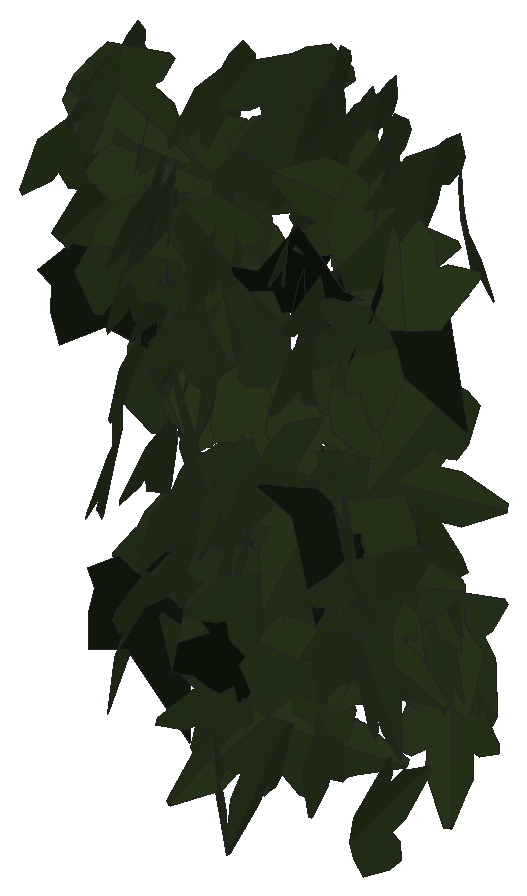
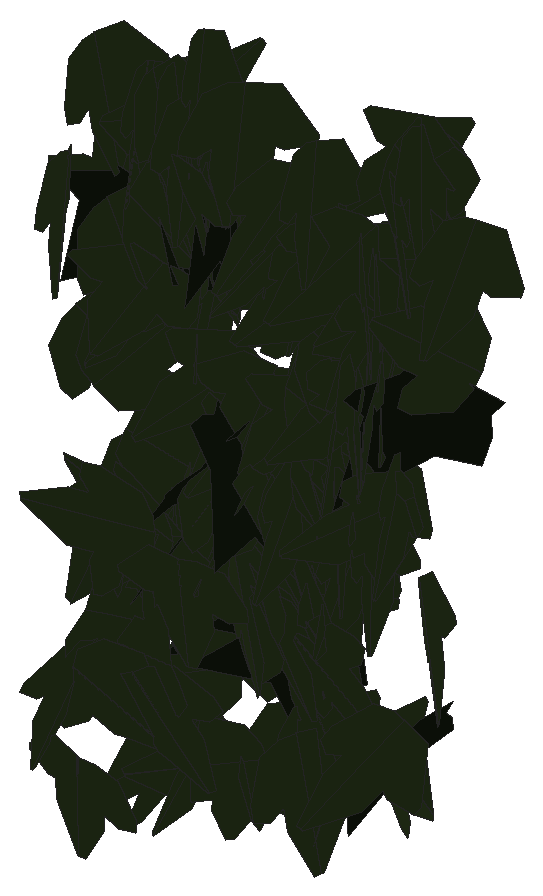
# SketchUp Ruby script. Lengths in inches.
U = 1.inch
M = Sketchup.active_model
def pt(a) = Geom::Point3d.new(a.map { |v| v * U })
def face(e, loops, mat)
  f = e.add_face(loops[0].map { |a| pt(a) })
  loops[1..].each { |l| e.add_face(l.map { |a| pt(a) }).erase! }
  f.material = f.back_material = mat if mat
  f
end
# faces: each face lists its corners as indices into pts; further lists are holes
def faces(e, pts, list, mat = nil) = list.each { |f| face(e, (f[0].is_a?(Array) ? f : [f]).map { |l| l.map { |i| pts[i] } }, mat) }
# xy, xz, yz: faces in a plane at the given z, y or x. An outline is a flat list of corners, or four numbers for a rectangle; further outlines are holes
def ring(l) = l.size == 4 ? [[l[0], l[1]], [l[2], l[1]], [l[2], l[3]], [l[0], l[3]]] : l.each_slice(2).to_a
def flat(e, list, mat, &to3) = list.each { |f| face(e, (f[0].is_a?(Array) ? f : [f]).map { |l| ring(l).map { |u, v| to3.(u, v) } }, mat) }
def xy(e, z, list, mat = nil) = flat(e, list, mat) { |x, y| [x, y, z] }
def xz(e, y, list, mat = nil) = flat(e, list, mat) { |x, z| [x, y, z] }
def yz(e, x, list, mat = nil) = flat(e, list, mat) { |y, z| [x, y, z] }
def lines(e, pts, list) = list.each { |a, b| e.add_line(pt(pts[a]), pt(pts[b])) }
# prism: a flat outline (further loops are holes) pulled along v
def prism(e, loops, v, mat = nil)
  f = face(e, loops, mat); d = Geom::Vector3d.new(v.map { |x| x * U })
  f.pushpull(f.normal.samedirection?(d) ? d.length : -d.length)
end
def box(e, o, s, mat = nil) = prism(e, [[o, [o[0] + s[0], o[1], o[2]], [o[0] + s[0], o[1] + s[1], o[2]], [o[0], o[1] + s[1], o[2]]]], [0, 0, s[2]], mat)
def at(x, y, z, deg = 0) = Geom::Transformation.translation(pt([x, y, z])) * Geom::Transformation.rotation(ORIGIN, Z_AXIS, deg.degrees)
def axes(o, x, y, z) = Geom::Transformation.new([*x, 0, *y, 0, *z, 0, *pt(o).to_a, 1])
def part(name) = M.definitions.add(name)
# library, detail: a bought-in or finely detailed component or shape, given as its bounding box
def library(name, o, s) = part(name).tap { |d| box(d.entities, o, s) }
def detail(e, o, s) = box(e.add_group.entities, o, s)
def put(e, d, t, mat = nil) = e.add_instance(d, t).tap { |i| i.material = mat if mat }
def group(e, t, mat = nil) = e.add_group.tap { |g| g.transformation = t; g.material = mat if mat }.entities
root = M.entities
M.materials.add("efeu1").color = [18, 25, 13]
M.materials.add("efeu2").color = [43, 57, 29]
c1 = part("ivyleaf_10")
p = [[0,0.5,-0.03],[-0.0625,2.02,-0.43],[-0.19,2.01,-0.46],[-0.54,1.05,-0.29],[-0.52,0.625,-0.18],[-0.83,0.76,-0.28],
  [-1.16,0.64,-0.33],[-1.15,0.33,-0.24],[-0.77,-0.39,0.02],[-0.3,-0.51,0.16],[0.04,-0.48,0.23],[-0.02,2.01,-0.4375],
  [-0.06,2.01,-0.43],[0.04,-0.49,0.23],[0.67,-0.49,0.14],[1.38,0.36,-0.2],[1.375,0.51,-0.24],[0.81,0.65,-0.19],
  [0.62,0.59,-0.15],[0.6,1.09,-0.28],[0.5,1.23,-0.31]]
faces(c1.entities,p,[[0,1,2,3,4,5,6,7,8,9,10],[11,12,0,13,14,15,16,17,18,19,20]],"efeu2")
c2 = part("ivyleaf_9")
p = [[1.54,2.16,1.25],[1.36,2.04,1.19],[-0.21,0.99,0.68],[-0.71,1.11,0.82],[-0.85,0.86,0.67],[-0.8,0.17,0.21],
  [-0.9,-0.01,0.1],[-0.67,-0.16,-0.02],[-0.08,-0.08,-0.05],[-0.03,-0.6,-0.4],[0.65,-0.88,-0.66],[0.83,-0.6,-0.49],
  [1.29,-0.42,-0.43],[1.8125,-0.07,-0.26],[1.21,0.44,0.15]]
faces(c2.entities,p,[[0,1,2,3,4,5,6,7,8,9,10,11,12,13,14]],"efeu1")
put(root,c1,axes([15.69,224.67,212.67],[-0.32703,0.04705,-0.37528],[0.36424,-0.09447,-0.32925],[-0.10189,-0.48873,0.02752]))
put(root,c1,axes([17.4,224.73,209.52],[-0.28401,-0.4041,0.07775],[-0.03453,-0.07074,-0.49377],[0.41006,-0.28584,0.01228]))
put(root,c1,axes([17.71,224.51,208.98],[-0.17834,0.44878,0.12959],[-0.06198,0.11475,-0.48269],[-0.46298,-0.18823,0.0147]))
put(root,c1,axes([15.59,224.82,212.34],[0.34047,-0.08844,0.35533],[0.34165,-0.09782,-0.35172],[0.13173,0.4823,-0.00618]))
put(root,c1,axes([14.57,224.93,213.75],[-0.00712,-0.42389,0.26508],[0.02002,-0.26514,-0.42344],[0.49955,0.00458,0.02074]))
put(root,c1,axes([17.17,224.95,213.28],[0.05774,0.30499,0.39198],[-0.05921,-0.38757,0.31029],[0.49311,-0.08225,-0.00864]))
put(root,c1,axes([15.52,224.68,210.34],[-0.34059,0.36403,-0.03849],[-0.02663,0.0278,0.49852],[0.36509,0.34163,0.00045]))
put(root,c1,axes([15.72,224.64,211.7],[-0.30712,-0.37365,-0.12675],[0.08006,0.09827,-0.48367],[0.38635,-0.31738,-0.00053]))
put(root,c2,axes([16.62,224.86,212.12],[0.47976,0.0051,0.14073],[-0.14077,0.00386,0.47976],[0.00381,-0.49996,0.00514]))
put(root,c1,axes([15.85,225.01,207.53],[0.10161,0.23758,-0.42806],[-0.17663,-0.38994,-0.25835],[-0.45659,0.20372,0.00469]))
put(root,c1,axes([16.22,224.92,211.65],[-0.1968,0.36183,0.28346],[0.09291,-0.27067,0.41001],[0.45015,0.21405,0.0393]))
put(root,c1,axes([16.16,224.99,207.41],[0.0555,-0.41348,0.2756],[0.07978,-0.2663,-0.4156],[0.49046,0.0901,0.03642]))
put(root,c1,axes([15.58,224.87,207.32],[-0.23078,0.34048,-0.28429],[0.14441,-0.24533,-0.41105],[-0.41939,-0.27183,0.01489]))
put(root,c1,axes([16.85,224.9,212.35],[0.1218,-0.47391,0.10282],[0.02755,-0.09908,-0.48931],[0.48415,0.12486,0.00198]))
put(root,c1,axes([16.23,224.74,209.13],[-0.369,-0.33564,-0.0344],[0.02551,0.02307,-0.49882],[0.33643,-0.36988,0.00009]))
put(root,c1,axes([16.68,224.76,213.12],[0.18254,-0.45116,-0.11461],[-0.03577,0.10915,-0.48663],[0.46411,0.18585,0.00758]))
put(root,c1,axes([14.74,224.5,212.26],[-0.10997,-0.20497,-0.4426],[0.28357,0.34228,-0.22897],[0.39685,-0.30138,0.04097]))
put(root,c1,axes([17.5,224.75,212.03],[0.262,-0.05993,-0.42162],[-0.40198,0.12863,-0.26808],[0.1406,0.47944,0.01922]))
put(root,c1,axes([17.55,224.79,209.77],[-0.26676,-0.42196,-0.02812],[0.01178,0.02581,-0.49919],[0.42273,-0.26699,-0.00383]))
put(root,c1,axes([16.59,225.0625,209.98],[-0.18231,-0.37531,0.27551],[0.01999,-0.30192,-0.39805],[0.46515,-0.13412,0.12509]))
put(root,c1,axes([15.39,225.1,211.77],[0.00432,-0.40516,0.29297],[0.02127,-0.29256,-0.40491],[0.49953,0.01596,0.01471]))
put(root,c1,axes([14.93,224.75,212.6875],[0.06248,-0.45228,-0.20381],[-0.02297,0.20256,-0.45655],[0.49555,0.06641,0.00453]))
put(root,c1,axes([14.51,224.69,213.74],[0.27445,0.14345,0.39256],[0.30006,0.25928,-0.30453],[-0.29094,0.40273,0.05623]))
put(root,c1,axes([17.46,224.79,209.26],[-0.29293,-0.3859,-0.12358],[0.07373,0.09919,-0.48448],[0.39844,-0.30207,-0.0012]))
put(root,c1,axes([16.5,224.61,210.57],[-0.1537,-0.28624,-0.38005],[0.17843,0.33557,-0.3249],[0.44106,-0.2355,-0.00101]))
put(root,c1,axes([16.81,224.73,211.87],[0.02036,-0.43541,-0.24495],[0.05121,0.24568,-0.43246],[0.49695,-0.00747,0.0546]))
put(root,c1,axes([17.33,224.6,209.17],[-0.1121,-0.25986,-0.41219],[0.18747,0.3674,-0.28261],[0.44976,-0.21791,0.01506]))
put(root,c1,axes([15.46,224.8125,209.28],[-0.06846,-0.47014,-0.15582],[0.02355,0.15403,-0.4751],[0.49473,-0.07239,0.00106]))
put(root,c1,axes([15.87,225.1,208.98],[-0.22773,-0.29857,0.33014],[-0.18356,-0.27484,-0.37519],[0.40552,-0.29209,0.01557]))
put(root,c1,axes([15.76,225.15,210.17],[-0.003,-0.42019,0.27098],[0.03525,-0.27049,-0.41904],[0.49875,0.01659,0.03125]))
put(root,c1,axes([15.72,224.75,212.52],[0.06723,-0.4078,-0.28139],[0.05,0.2881,-0.40558],[0.49293,0.0264,0.07952]))
put(root,c1,axes([17.26,224.96,208.96],[-0.21019,0.00989,-0.45357],[0.43774,-0.12689,-0.20563],[-0.11918,-0.48353,0.04468]))
put(root,c2,axes([15.82,224.63,208.6],[0.08755,0.17473,-0.46022],[0.17695,0.42503,0.19503],[0.45937,-0.19703,0.01258]))
put(root,c1,axes([15.53,225.25,211.25],[0.11794,-0.3146,0.37029],[0.17053,-0.33001,-0.33469],[0.45499,0.20523,0.02945]))
put(root,c1,axes([14.47,224.88,213.86],[0.01321,-0.4734,-0.16036],[-0.01386,0.16,-0.47351],[0.49963,0.01696,-0.00889]))
put(root,c1,axes([14.05,224.8125,213.05],[-0.15257,-0.41022,-0.24175],[0.11842,0.21319,-0.4365],[0.46119,-0.19045,0.0321]))
put(root,c2,axes([16.62,225.27,210.18],[-0.00957,-0.48571,0.11831],[0.01016,-0.1185,-0.48565],[0.49981,-0.00689,0.01214]))
put(root,c1,axes([15.96,225.14,210.18],[-0.18422,-0.43462,0.16483],[-0.05822,-0.15433,-0.47201],[0.46116,-0.1931,0.00625]))
put(root,c1,axes([17.32,224.7,209.66],[-0.10025,0.17783,-0.45643],[-0.22465,0.39732,0.20414],[0.4353,0.246,0.00024]))
put(root,c1,axes([15.35,225.04,207.77],[-0.38819,-0.01723,0.31466],[0.31357,0.02858,0.3884],[-0.03137,0.49889,-0.01138]))
put(root,c1,axes([17.38,224.65,213.11],[0.04929,0.15498,-0.47281],[0.15081,0.44813,0.16261],[0.47416,-0.15864,-0.00256]))
put(root,c1,axes([16.41,224.86,208.54],[-0.22974,-0.1561,-0.41576],[0.37915,0.17479,-0.27513],[0.23123,-0.44168,0.03806]))
put(root,c1,axes([15.54,225.12,209.72],[-0.0086,-0.01299,0.49976],[0.49822,-0.04143,0.0075],[0.04121,0.49811,0.01366]))
put(root,c1,axes([15.22,224.85,209.6875],[-0.03202,-0.40208,-0.29548],[0.09154,0.28633,-0.39954],[0.49051,-0.07968,0.05527]))
put(root,c1,axes([16.63,225.06,213.61],[0.0493,-0.49566,-0.04353],[0.00159,0.0439,-0.49807],[0.49756,0.04897,0.0059]))
put(root,c1,axes([16.1,224.98,211.08],[0.39232,0.25302,0.17907],[0.1459,0.10412,-0.46677],[-0.27349,0.4185,0.00786]))
put(root,c1,axes([15.75,225.26,209.51],[0.09709,-0.43985,0.21704],[0.06999,-0.20656,-0.44993],[0.48546,0.11775,0.02146]))
put(root,c1,axes([14.83,224.98,212.54],[0.15615,-0.43201,-0.19745],[-0.03509,0.19678,-0.45831],[0.47369,0.15698,0.03113]))
put(root,c1,axes([17.28,225.13,209.01],[0.4742,0.02406,-0.15671],[-0.1565,-0.00817,-0.47481],[-0.02541,0.49935,-0.00022]))
put(root,c1,axes([14.68,224.96,211.91],[0.09842,-0.43653,-0.22306],[0.03343,0.23296,-0.44115],[0.48908,0.07192,0.07505]))
put(root,c1,axes([14.4,225.34,208.11],[0.17728,-0.3616,0.29634],[0.14653,-0.25799,-0.40245],[0.44396,0.22954,0.01449]))
put(root,c1,axes([17.65,225.02,212.48],[0.44746,0.2184,0.04562],[-0.04613,-0.00947,0.49778],[0.2183,-0.44968,0.01168]))
put(root,c1,axes([15.01,225.07,210.72],[-0.09778,-0.0284,0.48952],[0.47947,0.09901,0.10152],[-0.1027,0.48928,0.00787]))
put(root,c1,axes([14.375,224.97,212.92],[0.07465,0.00152,0.49439],[0.42936,0.24769,-0.06559],[-0.24511,0.43434,0.03567]))
put(root,c1,axes([14.79,224.89,212.21],[-0.17607,-0.31937,-0.34205],[0.15411,0.30551,-0.36458],[0.44187,-0.23381,-0.00915]))
put(root,c2,axes([16.8,225.32,209.46],[0.18169,-0.46006,0.07303],[0.0192,-0.07092,-0.49457],[0.46543,0.18252,-0.0081]))
put(root,c1,axes([15.65,225.12,209.42],[0.35609,-0.32111,-0.14173],[-0.09767,0.10327,-0.47937],[0.33713,0.36909,0.01082]))
put(root,c1,axes([14.9375,225.06,212.75],[0.16656,-0.43658,-0.17791],[-0.02813,0.17914,-0.46596],[0.4706,0.16523,0.03511]))
put(root,c1,axes([15.54,224.95,210.96],[0.24149,0.24447,0.3632],[0.26237,0.25125,-0.34356],[-0.35049,0.35652,-0.00693]))
put(root,c2,axes([16.77,224.8,212.72],[-0.07265,0.1026,-0.48394],[-0.39643,0.28051,0.11898],[0.29591,0.40098,0.04059]))
put(root,c2,axes([17.39,225.14,212.46],[-0.12477,-0.20083,-0.44057],[0.32007,0.30717,-0.23066],[0.3633,-0.33958,0.05191]))
put(root,c1,axes([15.55,225.22,207.61],[-0.21958,-0.44561,0.05673],[-0.0181,-0.05432,-0.49671],[0.44884,-0.22019,0.00772]))
put(root,c1,axes([17.7,225.41,211.27],[-0.22356,-0.31257,0.31987],[-0.08276,-0.32252,-0.373],[0.43951,-0.21972,0.09247]))
put(root,c1,axes([14.95,224.8,212.07],[0.07045,-0.08245,0.4881],[-0.10668,0.4789,0.0963],[-0.48338,-0.11771,0.04988]))
put(root,c1,axes([15.875,225.22,209.12],[0.4472,-0.2164,-0.05643],[-0.05069,0.02478,-0.49681],[0.21782,0.45006,0.00023]))
put(root,c1,axes([16,225.01,210.59],[0.20737,-0.12128,-0.43851],[-0.33163,0.28963,-0.23693],[0.31148,0.38911,0.03968]))
put(root,c1,axes([16.76,225.11,213.58],[0.19104,-0.42873,-0.17233],[-0.04139,0.16985,-0.46844],[0.46021,0.19324,0.0294]))
put(root,c1,axes([17.2,225.2,210.22],[0.17982,0.06656,-0.46177],[-0.46652,0.03074,-0.17724],[0.0048,0.4946,0.07316]))
put(root,c1,axes([17.26,225.24,209.37],[0.11827,-0.08712,-0.47794],[0.45522,-0.15193,0.14034],[-0.16968,-0.46833,0.04337]))
put(root,c1,axes([17.75,225.24,213.8],[-0.06138,-0.49597,0.01573],[-0.00022,-0.01583,-0.49975],[0.49622,-0.06135,0.00172]))
put(root,c1,axes([17.48,225.38,210.96],[-0.30119,-0.13207,-0.37662],[-0.34177,-0.1583,0.32884],[-0.2061,0.45552,0.00508]))
put(root,c1,axes([17.27,224.83,211.5],[0.00255,0.18225,0.46559],[0.02293,0.46507,-0.18217],[-0.49947,0.02228,-0.00599]))
put(root,c1,axes([17.06,224.82,211.68],[0.00246,0.05222,0.49726],[-0.00188,0.49726,-0.05221],[-0.49999,-0.00162,0.00265]))
put(root,c1,axes([15.85,225.24,208.99],[0.44796,-0.18191,-0.12744],[-0.11856,0.04675,-0.48348],[0.18781,0.46338,-0.00125]))
put(root,c1,axes([14.04,224.99,212.01],[0.0601,-0.35051,0.35147],[0.06068,0.35657,0.34522],[-0.49265,0.00116,0.08539]))
put(root,c1,axes([14.6,225.14,213.5],[0.28048,-0.34658,-0.22629],[-0.10346,0.20598,-0.4437],[0.40078,0.29572,0.04383]))
put(root,c1,axes([14.81,225.13,210.08],[0.04706,-0.44818,-0.21662],[-0.03394,0.21419,-0.45052],[0.49662,0.05711,-0.01026]))
put(root,c1,axes([17.45,225.39,212.35],[-0.13906,-0.46156,0.13277],[-0.02491,-0.1311,-0.48186],[0.47963,-0.14063,0.01347]))
put(root,c1,axes([15.14,224.96,211.3125],[-0.11075,-0.17749,-0.45413],[0.23026,0.39146,-0.20915],[0.42979,-0.25546,-0.00497]))
put(root,c2,axes([14.18,225.14,211.66],[-0.03737,-0.24165,-0.43613],[0.0953,0.42583,-0.24411],[0.48941,-0.10137,0.01423]))
put(root,c2,axes([17.24,224.9375,212.21],[-0.05376,0.20244,0.45401],[-0.10622,0.44144,-0.20941],[-0.48562,-0.11897,-0.00446]))
put(root,c1,axes([16.53,224.98,211.06],[0.11006,0.23341,0.42826],[0.16759,0.3942,-0.25791],[-0.45804,0.20032,0.00854]))
put(root,c1,axes([16.82,225.29,213.86],[0.03856,-0.49435,-0.06427],[0.00715,0.065,-0.4957],[0.49846,0.03731,0.01208]))
put(root,c1,axes([14.13,225.26,209.67],[0.20166,-0.42912,-0.15872],[-0.04903,0.15219,-0.47375],[0.45489,0.20664,0.0193]))
put(root,c1,axes([16.64,225.2,214.1875],[0.07931,-0.43994,-0.22396],[0.00856,0.22803,-0.44489],[0.4936,0.06674,0.0437]))
put(root,c2,axes([14.375,225.4,208.26],[0.10969,-0.46449,-0.14904],[-0.0225,0.14779,-0.47713],[0.4873,0.11138,0.01152]))
put(root,c1,axes([17.31,224.97,206.97],[0.05635,-0.08202,0.49],[-0.16859,0.46072,0.09651],[-0.46733,-0.1761,0.02427]))
put(root,c1,axes([15.3,225.21,212.5],[-0.28397,-0.18151,-0.36935],[0.34806,0.13351,-0.33321],[0.21959,-0.44635,0.05053]))
put(root,c1,axes([17.2,225.22,213.6875],[0.02193,-0.44831,-0.22031],[0.0409,0.22139,-0.44644],[0.49784,0.00156,0.04638]))
put(root,c1,axes([15.19,225.14,211],[0.12083,-0.32446,-0.36073],[-0.04108,0.36357,-0.34078],[0.48344,0.11199,0.0612]))
put(root,c1,axes([15.3125,225.3,208.79],[0.23823,-0.11467,-0.42438],[-0.38676,0.17477,-0.26433],[0.20896,0.45421,-0.00543]))
put(root,c1,axes([16.09,225.36,209.3],[0.15423,-0.46433,-0.103],[-0.03896,0.09558,-0.48923],[0.47402,0.15894,-0.00669]))
put(root,c1,axes([15.68,225.14,210.17],[-0.01465,-0.3481,-0.35863],[0.03263,0.35735,-0.34819],[0.49872,-0.03361,0.01225]))
put(root,c1,axes([14.83,225.31,211.67],[0.04794,-0.46923,-0.16589],[-0.01966,0.16474,-0.47167],[0.49731,0.05175,-0.00265]))
put(root,c1,axes([16.92,225.67,212.81],[0.05953,-0.37716,0.32282],[0.09069,-0.31139,-0.38054],[0.48809,0.10386,0.03133]))
put(root,c1,axes([14.94,225.28,212.97],[-0.29397,-0.21474,-0.34273],[0.3079,0.15592,-0.36178],[0.26226,-0.42376,0.04056]))
put(root,c1,axes([14.74,225.26,211.84],[0.27945,-0.30914,-0.2763],[-0.04677,0.30757,-0.39143],[0.41197,0.24461,0.14298]))
put(root,c1,axes([17.27,225.23,213.61],[0.14689,-0.29536,-0.37574],[-0.06311,0.37766,-0.32154],[0.47375,0.14189,0.07367]))
put(root,c1,axes([16.17,225.36,207.45],[-0.12055,-0.06386,-0.48103],[0.47393,0.09096,-0.13084],[0.10422,-0.48749,0.03861]))
put(root,c1,axes([15.02,225.36,210.49],[0.29887,-0.32614,-0.23304],[-0.06183,0.24969,-0.42875],[0.39605,0.2851,0.10892]))
put(root,c1,axes([14.4,225.28,210.78],[0.0661,-0.369,-0.33087],[-0.0051,0.33327,-0.3727],[0.49559,0.05265,0.04029]))
put(root,c1,axes([16.84,225.55,213.9],[0.02732,-0.49923,0.00467],[0.00105,-0.00462,-0.49998],[0.49925,0.02733,0.00079]))
put(root,c1,axes([15.71,225.26,213.18],[-0.14491,-0.31667,-0.35878],[0.17304,0.31483,-0.34777],[0.44616,-0.22495,0.01835]))
put(root,c1,axes([15.22,225.43,213.68],[-0.02086,-0.47778,-0.14591],[0.04026,0.14395,-0.47713],[0.49794,-0.03165,0.03246]))
put(root,c1,axes([16.62,225.4,213.61],[-0.06943,-0.45883,-0.18617],[0.01997,0.18524,-0.46399],[0.49475,-0.07187,-0.0074]))
put(root,c1,axes([16.53,225.22,208.18],[0.03603,-0.03614,-0.49739],[0.36877,0.33765,0.00218],[0.33572,-0.367,0.05098]))
put(root,c1,axes([15.99,225.5,214.03],[-0.29543,-0.39849,-0.06269],[0.05948,0.03382,-0.4953],[0.39898,-0.30011,0.02742]))
put(root,c1,axes([16.55,225.24,207.51],[0.05814,-0.27501,-0.41351],[0.07852,0.41618,-0.26575],[0.49036,-0.03404,0.09158]))
put(root,c1,axes([16.63,225.62,213.27],[0.47694,-0.14884,0.01936],[0.01846,-0.00583,-0.49963],[0.14895,0.4773,-0.00007]))
put(root,c2,axes([16.25,225.18,210.26],[-0.0291,0.34819,0.35766],[-0.01757,0.35733,-0.3493],[-0.49884,-0.03289,-0.00856]))
put(root,c1,axes([16.21,225.21,209.72],[0.0858,-0.07127,-0.4874],[-0.01269,0.49425,-0.07451],[0.49242,0.02515,0.08301]))
put(root,c1,axes([14.82,225.375,211.41],[0.0557,-0.13061,-0.47941],[-0.21718,0.4275,-0.1417],[0.44691,0.22403,-0.00911]))
put(root,c1,axes([14.46,225.39,210.57],[-0.03023,-0.13177,-0.48138],[0.32832,0.35796,-0.11861],[0.37589,-0.32326,0.06488]))
put(root,c1,axes([15.59,225.38,212.82],[0.15481,-0.16872,-0.44449],[0.13693,0.46347,-0.12823],[0.45529,-0.08203,0.1897]))
put(root,c1,axes([17.16,226.07,208.95],[0.06256,0.28355,-0.40705],[-0.06857,-0.40139,-0.29015],[-0.49131,0.09212,-0.01133]))
put(root,c1,axes([17.28,225.78,209.68],[-0.41493,0.2384,-0.14492],[0.12193,-0.07864,-0.47849],[-0.25093,-0.43241,0.00712]))
put(root,c1,axes([16.74,225.83,212.27],[0.33427,0.25557,0.27009],[0.21062,0.16917,-0.42074],[-0.30644,0.39505,0.00544]))
put(root,c1,axes([16.6,226,208.28],[0.43996,0.00298,-0.23754],[-0.23739,0.02427,-0.43938],[0.00891,0.4994,0.02278]))
put(root,c1,axes([16.33,226.14,208.76],[0.14602,-0.02151,0.47772],[0.4639,-0.11487,-0.14697],[0.11608,0.48615,-0.01359]))
put(root,c1,axes([17.75,225.82,212.89],[-0.32063,0.23643,0.30215],[-0.25019,0.16969,-0.39826],[-0.29086,-0.40658,0.00949]))
put(root,c1,axes([14.18,225.8,208.54],[-0.17192,-0.27321,-0.38184],[0.24649,0.29357,-0.32103],[0.39961,-0.29862,0.03374]))
put(root,c1,axes([17.14,226.17,208.34],[0.35409,0.05638,-0.34848],[-0.34307,-0.06137,-0.35852],[-0.0832,0.49301,-0.00477]))
put(root,c1,axes([16.12,226.15,209.66],[0.49083,0.08236,0.04797],[0.04708,0.00929,-0.49769],[-0.08287,0.49308,0.00137]))
put(root,c1,axes([16.84,226.07,209.88],[-0.01942,0.01345,-0.49944],[0.49883,-0.0276,-0.02014],[-0.02811,-0.49906,-0.01234]))
put(root,c1,axes([17.08,226.35,207.46],[0.4817,-0.03301,0.12989],[0.12981,-0.00565,-0.48282],[0.03335,0.49888,0.00312]))
put(root,c1,axes([17.29,226.16,208.4],[-0.05252,0.45729,0.19527],[-0.01672,0.19462,-0.46026],[-0.49695,-0.05488,-0.00516]))
